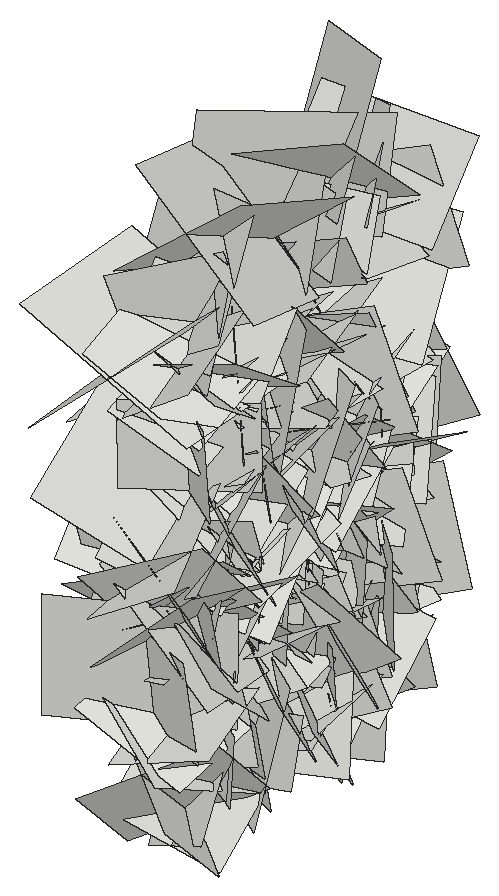
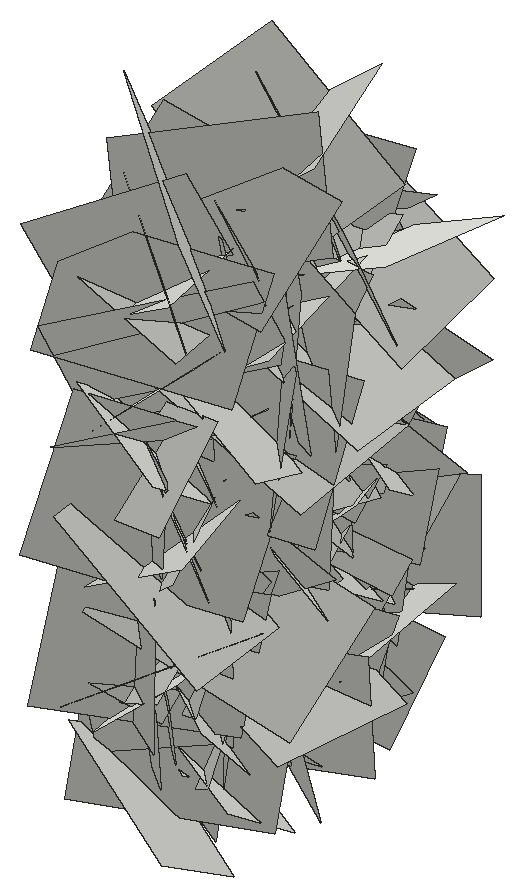
# SketchUp Ruby script. Lengths in inches.
U = 1.inch
M = Sketchup.active_model
def pt(a) = Geom::Point3d.new(a.map { |v| v * U })
def face(e, loops, mat)
  f = e.add_face(loops[0].map { |a| pt(a) })
  loops[1..].each { |l| e.add_face(l.map { |a| pt(a) }).erase! }
  f.material = f.back_material = mat if mat
  f
end
# faces: each face lists its corners as indices into pts; further lists are holes
def faces(e, pts, list, mat = nil) = list.each { |f| face(e, (f[0].is_a?(Array) ? f : [f]).map { |l| l.map { |i| pts[i] } }, mat) }
# xy, xz, yz: faces in a plane at the given z, y or x. An outline is a flat list of corners, or four numbers for a rectangle; further outlines are holes
def ring(l) = l.size == 4 ? [[l[0], l[1]], [l[2], l[1]], [l[2], l[3]], [l[0], l[3]]] : l.each_slice(2).to_a
def flat(e, list, mat, &to3) = list.each { |f| face(e, (f[0].is_a?(Array) ? f : [f]).map { |l| ring(l).map { |u, v| to3.(u, v) } }, mat) }
def xy(e, z, list, mat = nil) = flat(e, list, mat) { |x, y| [x, y, z] }
def xz(e, y, list, mat = nil) = flat(e, list, mat) { |x, z| [x, y, z] }
def yz(e, x, list, mat = nil) = flat(e, list, mat) { |y, z| [x, y, z] }
def lines(e, pts, list) = list.each { |a, b| e.add_line(pt(pts[a]), pt(pts[b])) }
# prism: a flat outline (further loops are holes) pulled along v
def prism(e, loops, v, mat = nil)
  f = face(e, loops, mat); d = Geom::Vector3d.new(v.map { |x| x * U })
  f.pushpull(f.normal.samedirection?(d) ? d.length : -d.length)
end
def box(e, o, s, mat = nil) = prism(e, [[o, [o[0] + s[0], o[1], o[2]], [o[0] + s[0], o[1] + s[1], o[2]], [o[0], o[1] + s[1], o[2]]]], [0, 0, s[2]], mat)
def at(x, y, z, deg = 0) = Geom::Transformation.translation(pt([x, y, z])) * Geom::Transformation.rotation(ORIGIN, Z_AXIS, deg.degrees)
def axes(o, x, y, z) = Geom::Transformation.new([*x, 0, *y, 0, *z, 0, *pt(o).to_a, 1])
def part(name) = M.definitions.add(name)
# library, detail: a bought-in or finely detailed component or shape, given as its bounding box
def library(name, o, s) = part(name).tap { |d| box(d.entities, o, s) }
def detail(e, o, s) = box(e.add_group.entities, o, s)
def put(e, d, t, mat = nil) = e.add_instance(d, t).tap { |i| i.material = mat if mat }
def group(e, t, mat = nil) = e.add_group.tap { |g| g.transformation = t; g.material = mat if mat }.entities
root = M.entities
c1 = part("Component\#6")
p = [[0.01,0,0],[0,3.24,4.54],[4.32,3.24,4.54],[4.33,0,0]]
faces(c1.entities,p,[[0,1,2,3]])
put(root,c1,axes([404.88,148.21,18.05],[-0.18781,1.38239,0.05917],[-0.11095,0.04609,-1.39025],[-1.46247,-0.18102,0.09787]))
put(root,c1,axes([404.88,151.36,16.73],[-0.05564,-1.33407,-0.12972],[-0.26745,-0.11766,1.31218],[-1.39538,0.07575,-0.24633]))
put(root,c1,axes([404.88,153.54,10.59],[-0.17173,1.22834,-0.55665],[-0.01226,-0.5619,-1.23655],[-1.42944,-0.14275,0.07748]))
put(root,c1,axes([404.88,150.02,13.53],[-0.11354,-0.10924,1.28227],[-0.18202,1.27641,0.09439],[-1.35193,-0.16268,-0.1204]))
put(root,c1,axes([404.88,150.46,17.01],[-0.04698,1.34267,-0.16756],[-0.13374,-0.17102,-1.33703],[-1.42802,-0.02815,0.13073]))
put(root,c1,axes([404.88,146.56,18.67],[-0.08115,0.67304,1.19325],[-0.03541,1.19384,-0.67552],[-1.45175,-0.06674,-0.05023]))
put(root,c1,axes([404.88,155.15,17.37],[-0.02517,0.60882,-1.16754],[-0.2041,-1.15679,-0.59929],[-1.38075,0.1599,0.10987]))
put(root,c1,axes([404.88,149.47,1.18],[-0.22795,-1.08393,0.44752],[-0.03192,0.45993,1.09954],[-1.24263,0.18702,-0.11034]))
put(root,c1,axes([404.88,145.22,20.96],[-0.20751,1.35949,-0.09859],[0.20583,-0.07077,-1.36145],[-1.43011,-0.20745,-0.18164]))
put(root,c1,axes([404.88,151.77,16.16],[-0.14743,1.12249,0.38129],[-0.0578,0.37744,-1.13105],[-1.25528,-0.14922,0.00729]))
put(root,c1,axes([404.88,155.16,12.125],[-0.20792,1.23942,0.0793],[0.14973,0.10203,-1.24521],[-1.30793,-0.18535,-0.15516]))
put(root,c1,axes([404.88,149.82,11.51],[-0.16938,-0.10345,1.35904],[0.25816,1.34416,0.13095],[-1.4215,0.25644,-0.13816]))
put(root,c1,axes([404.88,149.27,6.59],[0.15688,1.33929,-0.00269],[-0.18956,0.01708,-1.33541],[-1.40693,0.14704,0.17962]))
put(root,c1,axes([404.88,157.09,9.16],[-0.26081,-0.66319,-0.77037],[-0.09697,-0.77495,0.69635],[-1.07312,0.23121,0.12431]))
put(root,c1,axes([404.88,153.21,11.43],[0.14123,-0.96535,-0.93141],[-0.15435,-0.94087,0.95433],[-1.41351,0.00629,-0.19727]))
put(root,c1,axes([404.88,148.05,8.79],[-0.07068,0.0827,-1.14811],[-0.1221,-1.14474,-0.07576],[-1.21402,0.11031,0.07447]))
put(root,c1,axes([404.88,154.4,5.48],[0.14525,-0.2612,-1.20099],[-0.27145,-1.18798,0.22915],[-1.27422,0.2233,-0.18571]))
put(root,c1,axes([404.88,153.41,21.56],[-0.04666,0.60871,1.19242],[0.17987,1.18598,-0.59916],[-1.40769,0.13136,-0.11609]))
put(root,c1,axes([404.88,152.41,8.09],[0.02535,-1.06677,0.60381],[-0.0625,0.60222,1.06631],[-1.29785,-0.04984,-0.03955]))
put(root,c1,axes([404.88,151.84,12.71],[-0.09641,-0.969,-0.91768],[0.24854,-0.9171,0.94515],[-1.39265,-0.09659,0.2322]))
put(root,c1,axes([404.88,148.37,14.37],[-0.13394,0.02599,1.3483],[0.3112,1.32226,0.00203],[-1.39518,0.29244,-0.12899]))
put(root,c1,axes([404.88,148.8125,12.02],[-0.02959,0.36254,-1.01381],[-0.21176,-0.99828,-0.35148],[-1.12146,0.17893,0.09312]))
put(root,c1,axes([404.88,153.72,24.55],[0.10736,0.8301,-0.78481],[-0.26067,-0.75358,-0.8288],[-1.18252,0.24148,0.11144]))
put(root,c1,axes([404.88,144.59,11.1],[-0.20686,0.83944,0.54314],[-0.00436,0.55271,-0.85571],[-1.05982,-0.16612,-0.10249]))
put(root,c1,axes([404.88,150.33,13.2],[0.24126,0.02501,1.36725],[-0.05252,1.3853,-0.01709],[-1.44858,-0.04606,0.22834]))
put(root,c1,axes([404.88,153.16,13.74],[-0.07693,-1.07175,0.44962],[0.07215,0.4458,1.07364],[-1.22986,0.09319,0.03486]))
put(root,c1,axes([400.91,155.94,6.59],[-0.14653,0.65267,0.04592],[-0.0729,0.03218,-0.6644],[0.6897,0.14207,-0.06047]))
put(root,c1,axes([404.88,147.25,11.15],[-0.01251,0.83252,-0.66438],[-0.16644,-0.65852,-0.82239],[-1.1167,0.08883,0.13002]))
put(root,c1,axes([404.88,157.5,5.99],[-0.02733,0.34478,-1.12821],[0.04378,-1.12752,-0.34552],[-1.24973,-0.04704,0.01257]))
put(root,c1,axes([404.88,159.05,4.5],[-0.22831,-0.97739,-0.02602],[0.01319,-0.02938,1.00067],[-1.03632,0.21495,0.01847]))
put(root,c1,axes([404.88,156.09,10.89],[-0.02844,-1.01096,-0.23497],[-0.17327,-0.228,0.99963],[-1.08645,0.06282,-0.15327]))
put(root,c1,axes([404.88,158.38,15.93],[0.03304,0.59909,-1.16183],[0.1621,-1.15585,-0.5919],[-1.37611,-0.12177,-0.09762]))
put(root,c1,axes([404.88,147.43,1.76],[-0.0449,0.15818,1.07958],[-0.0304,1.07985,-0.15935],[-1.15617,-0.03454,-0.03773]))
put(root,c1,axes([404.88,156.6875,24.44],[-0.16473,0.01802,-1.18121],[0.23771,-1.16927,-0.04735],[-1.22945,-0.22849,0.14911]))
put(root,c1,axes([400.91,148.65,3.04],[-0.12439,-0.47488,0.46679],[-0.05284,0.47892,0.47469],[0.70386,-0.04797,0.11813]))
put(root,c1,axes([400.91,150.18,6.375],[-0.17639,-0.58204,-0.33942],[0.00316,-0.35025,0.59915],[0.71419,-0.1422,-0.08648]))
put(root,c1,axes([404.88,151.75,19.45],[-0.16935,0.44212,0.83371],[-0.05466,0.84022,-0.45546],[-0.99881,-0.12095,-0.11643]))
put(root,c1,axes([404.88,152.08,1.74],[-0.04493,0.85391,0.54577],[-0.09586,0.54089,-0.85328],[-1.06994,-0.08432,0.05353]))
put(root,c1,axes([404.88,158.83,13.98],[-0.00743,-1.2386,0.03478],[0.17851,0.0335,1.22715],[-1.30124,0.01167,0.16814]))
put(root,c1,axes([404.88,148.93,-0.125],[0.17085,0.2332,1.25619],[0.02467,1.2654,-0.2379],[-1.35409,0.05247,0.15416]))
put(root,c1,axes([404.88,148.09,7.11],[0.15706,0.67864,1.02073],[-0.03183,1.02986,-0.68036],[-1.29889,0.05683,0.1401]))
put(root,c1,axes([404.88,145.87,3.84],[-0.08046,-0.07863,0.91675],[-0.19442,0.90269,0.06223],[-0.95574,-0.17701,-0.08983]))
put(root,c1,axes([404.88,155.4,17.52],[0.19723,0.3027,-1.19403],[-0.0763,-1.20284,-0.31615],[-1.30348,0.11621,-0.16216]))
put(root,c1,axes([404.88,148.31,17.26],[-0.09379,0.98835,0.28145],[0.01751,0.28383,-0.99149],[-1.08916,-0.08054,-0.04018]))
put(root,c1,axes([404.88,151.01,19.39],[-0.01021,0.65154,-0.69294],[-0.23408,-0.67557,-0.63214],[-0.98066,0.15447,0.1581]))
put(root,c1,axes([404.88,157.43,12.97],[0.1074,-0.05602,-1.35571],[0.22854,-1.34155,0.07155],[-1.42001,-0.22014,-0.09102]))
put(root,c1,axes([400.91,152.72,13.34],[-0.14332,-0.62648,-0.12325],[0.10799,-0.14554,0.62801],[0.66813,-0.11086,-0.12794]))
put(root,c1,axes([404.88,154.9,1.8],[-0.03269,0.90387,0.50014],[-0.00572,0.50021,-0.90434],[-1.09498,-0.0296,-0.01021]))
put(root,c1,axes([400.91,149.02,5.32],[-0.19432,-0.67994,0.40742],[-0.04988,0.42677,0.69106],[0.83874,-0.13215,0.13549]))
put(root,c1,axes([404.88,160.22,19.0625],[0.13961,-0.68099,-1.03193],[0.07146,-1.03227,0.68982],[-1.30861,-0.12902,-0.07242]))
put(root,c1,axes([404.88,157.74,11.21],[-0.0595,-0.6331,0.72554],[-0.06262,0.72766,0.63038],[-1.01877,-0.00775,-0.08112]))
put(root,c1,axes([400.91,146,16.15],[-0.10062,0.63244,0.10884],[0.07256,0.11937,-0.63396],[0.67636,0.08128,0.0842]))
put(root,c1,axes([400.91,147.25,18.09],[-0.11506,-0.20062,0.68841],[-0.02156,0.69683,0.19986],[0.75976,-0.01061,0.10993]))
put(root,c1,axes([400.91,155.37,8.05],[-0.03179,-0.04018,0.69029],[-0.07893,0.6871,0.03676],[0.72868,0.07267,0.03409]))
put(root,c1,axes([400.91,151.91,13.09],[-0.06029,-0.61389,0.14039],[0.0496,0.13645,0.61563],[0.66568,-0.06576,-0.03315]))
put(root,c1,axes([404.88,153.47,7.93],[0.25077,0.36385,-1.26635],[0.08689,-1.28818,-0.35481],[-1.39394,-0.01484,-0.24993]))
put(root,c1,axes([404.88,158.45,22.43],[0.19892,0.24365,-1.12098],[-0.08242,-1.13056,-0.25875],[-1.21318,0.11676,-0.16622]))
put(root,c1,axes([400.91,151.13,9.12],[-0.15296,0.67587,0.31221],[0.03502,0.32352,-0.68509],[0.78839,0.11676,0.09101]))
put(root,c1,axes([404.88,148.76,4.0625],[-0.10183,-0.75916,-0.2873],[-0.20096,-0.26032,0.75126],[-0.83661,0.15493,-0.14549]))
put(root,c1,axes([404.88,155.05,20.66],[-0.11898,0.43702,0.87755],[0.10329,0.88388,-0.42771],[-1.03402,0.038,-0.1437]))
put(root,c1,axes([404.88,154.79,8.7],[0.06507,0.61236,-0.89404],[0.03144,-0.89608,-0.61173],[-1.14823,0.01016,-0.06741]))
put(root,c1,axes([400.91,151.99,2.12],[-0.1775,0.68354,0.35821],[0.06031,0.37649,-0.69181],[0.81579,0.12089,0.12909]))
put(root,c1,axes([400.91,151.79,4.27],[-0.00282,-0.67031,0.14172],[-0.04158,0.14164,0.66918],[0.72504,0.00552,0.03892]))
put(root,c1,axes([400.91,147.62,1.41],[-0.08717,-0.06025,0.7019],[0.04865,0.70471,0.06586],[0.74517,-0.05306,0.07781]))
put(root,c1,axes([400.91,156.87,7.65],[0.00449,0.50233,-0.39291],[0.02578,-0.39276,-0.50188],[0.67552,0.01165,0.02176]))
put(root,c1,axes([400.91,153.92,20.8125],[0.01755,0.277,-0.54123],[0.05617,-0.54003,-0.27476],[0.64202,0.03967,0.03883]))
put(root,c1,axes([404.88,152.6,3.91],[-0.02426,0.68313,0.69515],[0.0107,0.69547,-0.68312],[-1.03305,-0.00884,-0.0234]))
put(root,c1,axes([400.91,147.13,6.96],[-0.04816,-0.19283,0.63159],[0.07038,0.62854,0.19668],[0.69645,-0.07685,0.0238]))
put(root,c1,axes([404.88,158.68,8.63],[0.07829,-0.94373,0.27717],[-0.10215,0.26967,0.94388],[-1.03759,-0.09775,-0.07202]))
put(root,c1,axes([404.88,152.91,14.99],[0.05042,0.65822,-0.8803],[0.11398,-0.87969,-0.65195],[-1.15954,-0.05785,-0.10236]))
put(root,c1,axes([404.88,159.16,9.85],[0.13765,0.1916,-1.18129],[0.14512,-1.1828,-0.17679],[-1.2602,-0.11528,-0.14939]))
put(root,c1,axes([404.88,157.06,14.03],[0.04606,-0.47436,-0.98882],[0.12961,-0.98133,0.47614],[-1.15527,-0.12901,0.01399]))
put(root,c1,axes([404.88,149.64,15.49],[0.05397,-0.71515,0.49033],[-0.26351,0.45852,0.69456],[-0.88054,-0.18105,-0.1778]))
put(root,c1,axes([400.91,148.39,13.69],[0.056,0.56116,0.2115],[0.06403,0.20626,-0.56234],[0.63244,-0.07057,0.03821]))
put(root,c1,axes([404.88,147.71,9.53],[0.0202,0.73421,-0.62443],[-0.01239,-0.62433,-0.73445],[-1.02159,0.02209,-0.00344]))
put(root,c1,axes([400.91,146.72,8.375],[0.05548,0.31048,0.67068],[-0.12303,0.66747,-0.29994],[0.77368,0.08387,-0.09579]))
put(root,c1,axes([404.88,152.28,1.18],[0.22482,-0.75958,0.923],[0.06114,0.94282,0.76264],[-1.2656,-0.08938,0.2008]))
put(root,c1,axes([404.88,154.73,4.99],[0.23466,-0.21907,1.02966],[-0.17179,1.03255,0.25453],[-1.10257,-0.20751,0.17949]))
put(root,c1,axes([400.91,148.44,10.1],[0.02371,0.59128,0.15103],[0.13632,0.14317,-0.57956],[0.63236,-0.05303,0.11928]))
put(root,c1,axes([400.91,154.81,5.31],[0.03271,-0.68931,-0.29186],[-0.0897,-0.29345,0.68411],[0.78838,-0.00479,0.08995]))
put(root,c1,axes([400.91,155.07,5.6],[-0.26442,-0.95782,0.42161],[-0.12666,0.45666,0.96674],[1.10204,-0.17733,0.21227]))
put(root,c1,axes([404.88,146.38,17.95],[-0.09245,0.38694,0.78979],[0.04684,0.79459,-0.38441],[-0.93107,0.00155,-0.09776]))
put(root,c1,axes([400.91,155.43,2.74],[0.05213,0.12024,0.7107],[-0.06472,0.71048,-0.11598],[0.7613,0.05216,-0.05853]))
put(root,c1,axes([404.88,149.03,14.67],[0.12882,0.64149,-0.81464],[-0.00451,-0.8199,-0.64626],[-1.09909,0.07855,-0.09282]))
put(root,c1,axes([400.91,145.53,10.42],[-0.22479,1.04725,-0.16356],[-0.16331,-0.19548,-1.05191],[1.11161,0.18306,-0.18761]))
put(root,c1,axes([404.88,147.21,13.43],[0.06341,1.09172,0.23851],[0.19798,0.22572,-1.08003],[-1.16785,0.09755,-0.17015]))
put(root,c1,axes([400.91,146.09,12.1875],[-0.18427,0.52878,-0.65011],[0.11203,-0.64482,-0.55274],[0.8812,0.19255,-0.06567]))
put(root,c1,axes([404.88,151.57,3.27],[-0.14157,0.02397,-0.74069],[-0.04702,-0.75154,-0.01632],[-0.78414,0.04073,0.1347]))
put(root,c1,axes([400.91,154.48,3.89],[0.11783,0.23417,0.69133],[-0.11259,0.69704,-0.21902],[0.76547,0.06648,-0.13863]))
put(root,c1,axes([400.91,152.53,7.1875],[0.08757,-0.64703,0.3684],[-0.09594,0.35919,0.65114],[0.78338,0.11632,0.03856]))
put(root,c1,axes([404.88,153.68,-0.24],[-0.08313,-0.05331,0.78078],[-0.05564,0.78328,0.04821],[-0.82769,-0.0473,-0.08166]))
put(root,c1,axes([400.91,155.23,10.47],[-0.04155,0.12694,-0.87349],[-0.11983,-0.86787,-0.12105],[0.92792,-0.10639,-0.05475]))
put(root,c1,axes([404.88,154.93,13.48],[0.13332,0.92748,-0.67904],[0.1887,-0.69057,-0.91025],[-1.20375,-0.00553,-0.2179]))
put(root,c1,axes([404.88,152.46,19.1],[0.24316,-1.11668,0.32256],[0.08367,0.34299,1.13127],[-1.22923,-0.19755,0.14081]))
put(root,c1,axes([404.88,149.625,17.57],[-0.05592,-0.7816,-0.40589],[0.0657,-0.4089,0.77935],[-0.93124,0.01809,0.07936]))
put(root,c1,axes([400.91,153.02,6.56],[0.04835,0.51462,-0.41299],[0.10228,-0.41473,-0.50612],[0.69191,0.02534,0.10368]))
put(root,c1,axes([400.91,155.74,21.65],[-0.00825,-0.17983,-0.66547],[0.14401,-0.65286,0.17483],[0.71636,0.12918,-0.04281]))
put(root,c1,axes([404.88,147.06,-0.97],[-0.01135,-0.66277,0.66685],[0.09721,0.66298,0.66039],[-0.99185,0.07256,0.05709]))
put(root,c1,axes([400.91,154.86,6.54],[-0.11481,0.21277,-0.79232],[0.09254,-0.79167,-0.22453],[0.86468,0.11298,-0.08117]))
put(root,c1,axes([404.88,155.95,10.68],[-0.04823,-0.00518,0.84226],[0.02844,0.84305,0.00663],[-0.89236,0.02715,-0.04531]))
put(root,c1,axes([404.88,146.53,12.92],[-0.03124,-0.05121,0.8385],[0.00373,0.839,0.05136],[-0.89046,0.00531,-0.0292]))
put(root,c1,axes([404.88,152.8,10.75],[0.04843,-0.82009,-0.82841],[0.32646,-0.79109,0.80013],[-1.19171,-0.25004,0.18553]))
put(root,c1,axes([400.91,155.82,10.86],[-0.10869,-0.77244,0.23734],[0.13092,0.22145,0.77409],[0.8465,-0.13343,-0.08925]))
put(root,c1,axes([400.91,156.49,11.61],[-0.16435,-0.92659,-0.48849],[-0.14398,-0.47186,0.93815],[1.10094,-0.20004,0.04977]))
put(root,c1,axes([404.88,153.88,7.81],[-0.12498,-0.19712,-0.75186],[0.05107,-0.76085,0.19192],[-0.82232,-0.01729,0.12619]))
put(root,c1,axes([400.91,154.72,7.86],[0.01434,-0.12328,-0.7123],[0.10241,-0.70572,0.12398],[0.75939,0.0975,-0.00327]))
put(root,c1,axes([404.88,155.22,14.18],[0.0107,0.67836,0.43703],[-0.08223,0.43585,-0.67474],[-0.8514,-0.03357,0.07066]))
put(root,c1,axes([400.91,152.55,8.85],[-0.17208,0.39932,0.93109],[-0.08126,0.93542,-0.41455],[1.07081,0.13515,0.11817]))
put(root,c1,axes([404.88,155.14,21.07],[0.01676,0.7943,-0.14622],[-0.08914,-0.14383,-0.79043],[-0.85145,0.03069,0.07988]))
put(root,c1,axes([400.91,158.76,13.54],[-0.17018,-0.33172,-0.9968],[-0.1229,-0.99662,0.35033],[1.10678,-0.16167,-0.11436]))
put(root,c1,axes([404.88,151.77,10.3],[-0.00621,-0.04081,-0.81439],[-0.02737,-0.814,0.04098],[-0.86391,0.02608,0.00455]))
put(root,c1,axes([404.88,149.67,1.32],[-0.10197,-0.47157,-0.58691],[0.00963,-0.59236,0.47447],[-0.798,0.05311,0.08072]))
put(root,c1,axes([400.91,154.27,5.56],[-0.10843,0.64197,-0.78685],[-0.13439,-0.79271,-0.63027],[1.06801,-0.03458,-0.15919]))
put(root,c1,axes([404.88,154.27,5.56],[0.10843,0.64197,-0.78685],[0.13439,-0.79271,-0.63027],[-1.06801,-0.03458,-0.15919]))
put(root,c1,axes([400.91,149.67,1.32],[0.10197,-0.47157,-0.58691],[-0.00963,-0.59236,0.47447],[0.798,0.05311,0.08072]))
put(root,c1,axes([400.91,151.77,10.3],[0.00621,-0.04081,-0.81439],[0.02737,-0.814,0.04098],[0.86391,0.02608,0.00455]))
put(root,c1,axes([404.88,158.76,13.54],[0.17018,-0.33172,-0.9968],[0.1229,-0.99662,0.35033],[-1.10678,-0.16167,-0.11436]))
put(root,c1,axes([400.91,155.14,21.07],[-0.01676,0.7943,-0.14622],[0.08914,-0.14383,-0.79043],[0.85145,0.03069,0.07988]))
put(root,c1,axes([404.88,152.55,8.85],[0.17208,0.39932,0.93109],[0.08126,0.93542,-0.41455],[-1.07081,0.13515,0.11817]))
put(root,c1,axes([400.91,155.22,14.18],[-0.0107,0.67836,0.43703],[0.08223,0.43585,-0.67474],[0.8514,-0.03357,0.07066]))
put(root,c1,axes([404.88,154.72,7.86],[-0.01434,-0.12328,-0.7123],[-0.10241,-0.70572,0.12398],[-0.75939,0.0975,-0.00327]))
put(root,c1,axes([400.91,153.88,7.81],[0.12498,-0.19712,-0.75186],[-0.05107,-0.76085,0.19192],[0.82232,-0.01729,0.12619]))
put(root,c1,axes([404.88,156.49,11.61],[0.16435,-0.92659,-0.48849],[0.14398,-0.47186,0.93815],[-1.10094,-0.20004,0.04977]))
put(root,c1,axes([404.88,155.82,10.86],[0.10869,-0.77244,0.23734],[-0.13092,0.22145,0.77409],[-0.8465,-0.13343,-0.08925]))
put(root,c1,axes([400.91,152.8,10.75],[-0.04843,-0.82009,-0.82841],[-0.32646,-0.79109,0.80013],[1.19171,-0.25004,0.18553]))
put(root,c1,axes([400.91,146.53,12.92],[0.03124,-0.05121,0.8385],[-0.00373,0.839,0.05136],[0.89046,0.00531,-0.0292]))
put(root,c1,axes([400.91,155.95,10.68],[0.04823,-0.00518,0.84226],[-0.02844,0.84305,0.00663],[0.89236,0.02715,-0.04531]))
put(root,c1,axes([404.88,154.86,6.54],[0.11481,0.21277,-0.79232],[-0.09254,-0.79167,-0.22453],[-0.86468,0.11298,-0.08117]))
put(root,c1,axes([400.91,147.06,-0.97],[0.01135,-0.66277,0.66685],[-0.09721,0.66298,0.66039],[0.99185,0.07256,0.05709]))
put(root,c1,axes([404.88,155.74,21.65],[0.00825,-0.17983,-0.66547],[-0.14401,-0.65286,0.17483],[-0.71636,0.12918,-0.04281]))
put(root,c1,axes([404.88,153.02,6.56],[-0.04835,0.51462,-0.41299],[-0.10228,-0.41473,-0.50612],[-0.69191,0.02534,0.10368]))
put(root,c1,axes([400.91,149.625,17.57],[0.05592,-0.7816,-0.40589],[-0.0657,-0.4089,0.77935],[0.93124,0.01809,0.07936]))
put(root,c1,axes([400.91,152.46,19.1],[-0.24316,-1.11668,0.32256],[-0.08367,0.34299,1.13127],[1.22923,-0.19755,0.14081]))
put(root,c1,axes([400.91,154.93,13.48],[-0.13332,0.92748,-0.67904],[-0.1887,-0.69057,-0.91025],[1.20375,-0.00553,-0.2179]))
put(root,c1,axes([404.88,155.23,10.47],[0.04155,0.12694,-0.87349],[0.11983,-0.86787,-0.12105],[-0.92792,-0.10639,-0.05475]))
put(root,c1,axes([400.91,153.68,-0.24],[0.08313,-0.05331,0.78078],[0.05564,0.78328,0.04821],[0.82769,-0.0473,-0.08166]))
put(root,c1,axes([404.88,152.53,7.1875],[-0.08757,-0.64703,0.3684],[0.09594,0.35919,0.65114],[-0.78338,0.11632,0.03856]))
put(root,c1,axes([404.88,154.48,3.89],[-0.11783,0.23417,0.69133],[0.11259,0.69704,-0.21902],[-0.76547,0.06648,-0.13863]))
put(root,c1,axes([400.91,151.57,3.27],[0.14157,0.02397,-0.74069],[0.04702,-0.75154,-0.01632],[0.78414,0.04073,0.1347]))
put(root,c1,axes([404.88,146.09,12.1875],[0.18427,0.52878,-0.65011],[-0.11203,-0.64482,-0.55274],[-0.8812,0.19255,-0.06567]))
put(root,c1,axes([400.91,147.21,13.43],[-0.06341,1.09172,0.23851],[-0.19798,0.22572,-1.08003],[1.16785,0.09755,-0.17015]))
put(root,c1,axes([404.88,145.53,10.42],[0.22479,1.04725,-0.16356],[0.16331,-0.19548,-1.05191],[-1.11161,0.18306,-0.18761]))
put(root,c1,axes([400.91,149.03,14.67],[-0.12882,0.64149,-0.81464],[0.00451,-0.8199,-0.64626],[1.09909,0.07855,-0.09282]))
put(root,c1,axes([404.88,155.43,2.74],[-0.05213,0.12024,0.7107],[0.06472,0.71048,-0.11598],[-0.7613,0.05216,-0.05853]))
put(root,c1,axes([400.91,146.38,17.95],[0.09245,0.38694,0.78979],[-0.04684,0.79459,-0.38441],[0.93107,0.00155,-0.09776]))
put(root,c1,axes([404.88,155.07,5.6],[0.26442,-0.95782,0.42161],[0.12666,0.45666,0.96674],[-1.10204,-0.17733,0.21227]))
put(root,c1,axes([404.88,154.81,5.31],[-0.03271,-0.68931,-0.29186],[0.0897,-0.29345,0.68411],[-0.78838,-0.00479,0.08995]))
put(root,c1,axes([404.88,148.44,10.1],[-0.02371,0.59128,0.15103],[-0.13632,0.14317,-0.57956],[-0.63236,-0.05303,0.11928]))
put(root,c1,axes([400.91,154.73,4.99],[-0.23466,-0.21907,1.02966],[0.17179,1.03255,0.25453],[1.10257,-0.20751,0.17949]))
put(root,c1,axes([400.91,152.28,1.18],[-0.22482,-0.75958,0.923],[-0.06114,0.94282,0.76264],[1.2656,-0.08938,0.2008]))
put(root,c1,axes([404.88,146.72,8.375],[-0.05548,0.31048,0.67068],[0.12303,0.66747,-0.29994],[-0.77368,0.08387,-0.09579]))
put(root,c1,axes([400.91,147.71,9.53],[-0.0202,0.73421,-0.62443],[0.01239,-0.62433,-0.73445],[1.02159,0.02209,-0.00344]))
put(root,c1,axes([404.88,148.39,13.69],[-0.056,0.56116,0.2115],[-0.06403,0.20626,-0.56234],[-0.63244,-0.07057,0.03821]))
put(root,c1,axes([400.91,149.64,15.49],[-0.05397,-0.71515,0.49033],[0.26351,0.45852,0.69456],[0.88054,-0.18105,-0.1778]))
put(root,c1,axes([400.91,157.06,14.03],[-0.04606,-0.47436,-0.98882],[-0.12961,-0.98133,0.47614],[1.15527,-0.12901,0.01399]))
put(root,c1,axes([400.91,159.16,9.85],[-0.13765,0.1916,-1.18129],[-0.14512,-1.1828,-0.17679],[1.2602,-0.11528,-0.14939]))
put(root,c1,axes([400.91,152.91,14.99],[-0.05042,0.65822,-0.8803],[-0.11398,-0.87969,-0.65195],[1.15954,-0.05785,-0.10236]))
put(root,c1,axes([400.91,158.68,8.63],[-0.07829,-0.94373,0.27717],[0.10215,0.26967,0.94388],[1.03759,-0.09775,-0.07202]))
put(root,c1,axes([404.88,147.13,6.96],[0.04816,-0.19283,0.63159],[-0.07038,0.62854,0.19668],[-0.69645,-0.07685,0.0238]))
put(root,c1,axes([400.91,152.6,3.91],[0.02426,0.68313,0.69515],[-0.0107,0.69547,-0.68312],[1.03305,-0.00884,-0.0234]))
put(root,c1,axes([404.88,153.92,20.8125],[-0.01755,0.277,-0.54123],[-0.05617,-0.54003,-0.27476],[-0.64202,0.03967,0.03883]))
put(root,c1,axes([404.88,156.87,7.65],[-0.00449,0.50233,-0.39291],[-0.02578,-0.39276,-0.50188],[-0.67552,0.01165,0.02176]))
put(root,c1,axes([404.88,147.62,1.41],[0.08717,-0.06025,0.7019],[-0.04865,0.70471,0.06586],[-0.74517,-0.05306,0.07781]))
put(root,c1,axes([404.88,151.79,4.27],[0.00282,-0.67031,0.14172],[0.04158,0.14164,0.66918],[-0.72504,0.00552,0.03892]))
put(root,c1,axes([404.88,151.99,2.12],[0.1775,0.68354,0.35821],[-0.06031,0.37649,-0.69181],[-0.81579,0.12089,0.12909]))
put(root,c1,axes([400.91,154.79,8.7],[-0.06507,0.61236,-0.89404],[-0.03144,-0.89608,-0.61173],[1.14823,0.01016,-0.06741]))
put(root,c1,axes([400.91,155.05,20.66],[0.11898,0.43702,0.87755],[-0.10329,0.88388,-0.42771],[1.03402,0.038,-0.1437]))
put(root,c1,axes([400.91,148.76,4.0625],[0.10183,-0.75916,-0.2873],[0.20096,-0.26032,0.75126],[0.83661,0.15493,-0.14549]))
